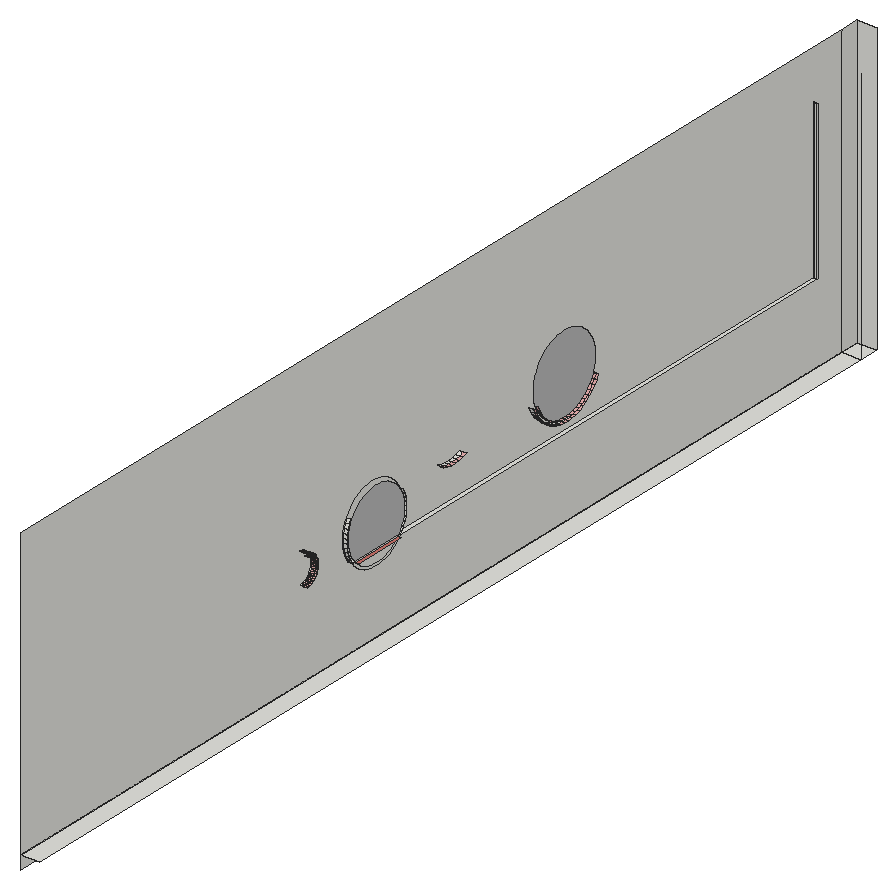
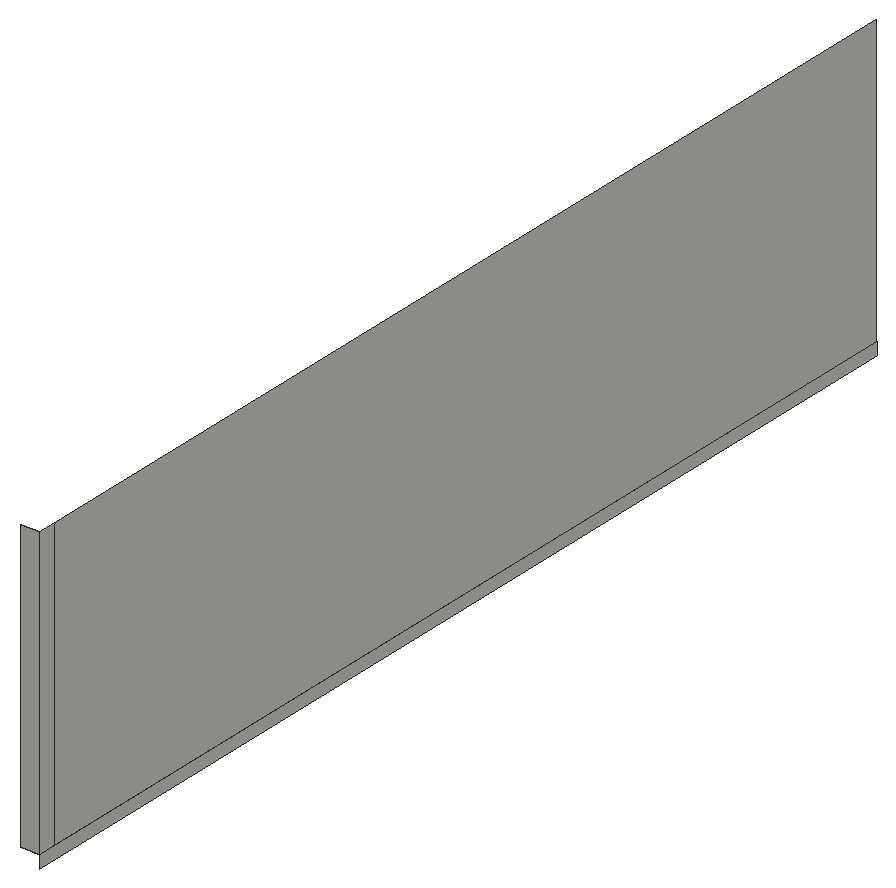
# SketchUp Ruby script. Lengths in inches.
U = 1.inch
M = Sketchup.active_model
def pt(a) = Geom::Point3d.new(a.map { |v| v * U })
def face(e, loops, mat)
  f = e.add_face(loops[0].map { |a| pt(a) })
  loops[1..].each { |l| e.add_face(l.map { |a| pt(a) }).erase! }
  f.material = f.back_material = mat if mat
  f
end
# faces: each face lists its corners as indices into pts; further lists are holes
def faces(e, pts, list, mat = nil) = list.each { |f| face(e, (f[0].is_a?(Array) ? f : [f]).map { |l| l.map { |i| pts[i] } }, mat) }
# xy, xz, yz: faces in a plane at the given z, y or x. An outline is a flat list of corners, or four numbers for a rectangle; further outlines are holes
def ring(l) = l.size == 4 ? [[l[0], l[1]], [l[2], l[1]], [l[2], l[3]], [l[0], l[3]]] : l.each_slice(2).to_a
def flat(e, list, mat, &to3) = list.each { |f| face(e, (f[0].is_a?(Array) ? f : [f]).map { |l| ring(l).map { |u, v| to3.(u, v) } }, mat) }
def xy(e, z, list, mat = nil) = flat(e, list, mat) { |x, y| [x, y, z] }
def xz(e, y, list, mat = nil) = flat(e, list, mat) { |x, z| [x, y, z] }
def yz(e, x, list, mat = nil) = flat(e, list, mat) { |y, z| [x, y, z] }
def lines(e, pts, list) = list.each { |a, b| e.add_line(pt(pts[a]), pt(pts[b])) }
# prism: a flat outline (further loops are holes) pulled along v
def prism(e, loops, v, mat = nil)
  f = face(e, loops, mat); d = Geom::Vector3d.new(v.map { |x| x * U })
  f.pushpull(f.normal.samedirection?(d) ? d.length : -d.length)
end
def box(e, o, s, mat = nil) = prism(e, [[o, [o[0] + s[0], o[1], o[2]], [o[0] + s[0], o[1] + s[1], o[2]], [o[0], o[1] + s[1], o[2]]]], [0, 0, s[2]], mat)
def at(x, y, z, deg = 0) = Geom::Transformation.translation(pt([x, y, z])) * Geom::Transformation.rotation(ORIGIN, Z_AXIS, deg.degrees)
def axes(o, x, y, z) = Geom::Transformation.new([*x, 0, *y, 0, *z, 0, *pt(o).to_a, 1])
def part(name) = M.definitions.add(name)
# library, detail: a bought-in or finely detailed component or shape, given as its bounding box
def library(name, o, s) = part(name).tap { |d| box(d.entities, o, s) }
def detail(e, o, s) = box(e.add_group.entities, o, s)
def put(e, d, t, mat = nil) = e.add_instance(d, t).tap { |i| i.material = mat if mat }
def group(e, t, mat = nil) = e.add_group.tap { |g| g.transformation = t; g.material = mat if mat }.entities
root = M.entities
M.materials.add("Generic").color = [224, 169, 169]
M.materials.add("[Mirror 01]").color = [185, 185, 185]
M.materials.add("[Wood Floor Dark]").color = [198, 114, 106]
xy(root,0,[[0,0.4375,9,481.125],[0,481.125,9,490.125]])
xy(root,46.5,[[9,181.21,10.6875,181.21,10.6875,196.98,9,198.375],[10.6875,196.98,10.6875,209.04,9,209.04,9,198.375],[9,209.04,10.6875,453.375],[9,453.375,10.6875,453.625]])
xy(root,46.5,[[10.6875,182.81,12.375,207.45]],"[Wood Floor Dark]")
xz(root,453.375,[[9,46.5,10.6875,120]])
xz(root,453.625,[[9,46.5,10.6875,120]])
xz(root,490.125,[[0,0,9,135.25]])
yz(root,0,[[0,-6,490.125,0],[0.4375,0,481.125,135.25],[481.125,0,490.125,135.25]])
yz(root,9,[[181.21,46.5,209.04,46.5,209.84,47.59,210.84,49.33,211.63,51.17,212.21,53.09,212.56,55.07,212.6875,57.07,212.58,59.07,212.25,61.05,211.7,62.97,210.93,64.82,209.95,66.58,208.78,68.2,207.4375,69.69,205.93,71.01,204.28,72.15,202.51,73.1,200.65,73.84,198.71,74.36,196.73,74.65,194.73,74.72,192.73,74.5625,190.76,74.18,188.85,73.57,187.02,72.74,185.3,71.72,183.7,70.5,182.26,69.11,180.98,67.57,179.89,65.89,178.99,64.1,178.31,62.21,177.84,60.26,177.6,58.27,177.59,56.27,177.81,54.27,178.25,52.32,178.91,50.42,179.79,48.62,180.86,46.93],[453.375,46.5,453.625,120]])
yz(root,10.6875,[[194.52,39.62,196.53,39.66,198.52,39.9375,200.46,40.4375,202.33,41.15,204.11,42.08,205.77,43.2,207.29,44.5,208.66,45.97,209.04,46.5,207.45,46.5,206.43,45.4,205.01,44.19,203.47,43.15,201.82,42.29,200.08,41.625,198.27,41.16,196.43,40.91,194.57,40.86,192.71,41.03,190.89,41.41,189.12,42,187.43,42.78,185.84,43.75,184.375,44.9,183.05,46.21,182.81,46.5,181.21,46.5,182.12,45.37,183.55,43.96,185.13,42.73,186.84,41.68,188.66,40.84,190.57,40.21,192.53,39.8],[194.57,40.86,196.43,40.91,198.27,41.16,200.08,41.625,201.82,42.29,203.47,43.15,205.01,44.19,206.43,45.4,207.45,46.5,182.81,46.5,183.05,46.21,184.375,44.9,185.84,43.75,187.43,42.78,189.12,42,190.89,41.41,192.71,41.03],[453.375,46.5,453.625,120]])
yz(root,10.6875,[[182.81,46.5,207.45,46.5,207.7,46.77,208.8,48.27,209.72,49.89,210.46,51.6,210.99,53.38,211.32,55.22,211.4375,57.07,211.34,58.93,211.04,60.77,210.52,62.5625,209.81,64.28,208.9,65.91,207.8125,67.42,206.5625,68.8,205.16,70.03,203.63,71.09,201.99,71.97,200.26,72.65,198.46,73.14,196.62,73.41,194.75,73.48,192.9,73.33,191.07,72.97,189.3,72.4,187.6,71.64,186,70.69,184.52,69.56,183.17,68.27,181.98,66.83,180.97,65.27,180.14,63.6,179.5,61.85,179.07,60.04,178.85,58.19,178.84,56.33,179.04,54.48,179.45,52.66,180.06,50.9,180.875,49.23,181.875,47.65],[305.93,53.75,307.99,53.95,310.02,54.375,311.98,55.03,313.86,55.9,315.62,56.99,317.25,58.26,318.72,59.72,320.02,61.33,321.12,63.08,322.02,64.94,322.7,66.9,323.15,68.92,323.375,70.97,323.36,73.04,323.11,75.1,322.62,77.11,321.91,79.05,320.98,80.9,319.85,82.64,318.53,84.23,317.03,85.66,315.38,86.91,313.6,87.96,311.71,88.81,309.74,89.43,307.71,89.83,305.64,89.99,303.58,89.91,301.53,89.6,299.53,89.06,297.61,88.29,295.79,87.3125,294.09,86.13,292.54,84.76,291.15,83.23,289.95,81.54,288.94,79.73,288.15,77.82,287.58,75.83,287.25,73.79,287.15,71.72,287.28,69.66,287.65,67.62,288.25,65.64,289.07,63.74,290.1,61.95,291.33,60.28,292.74,58.77,294.32,57.43,296.03,56.27,297.87,55.32,299.81,54.58,301.8125,54.07,303.86,53.8]],"[Mirror 01]")
p = [[10.6875,180.86,46.93],[10.6875,181.21,46.5],[9,181.21,46.5],[9,180.86,46.93],[10.6875,209.04,46.5],[10.6875,209.84,47.59],
  [9,209.84,47.59],[9,209.04,46.5],[10.6875,179.79,48.62],[9,179.79,48.62],[10.6875,210.84,49.33],[9,210.84,49.33],
  [10.6875,178.91,50.42],[9,178.91,50.42],[10.6875,152.83,49.33],[10.6875,153.61,49.5],[9,153.61,49.5],[9,152.83,49.33],
  [12.375,153.61,49.5],[12.375,152.83,49.33],[10.6875,211.63,51.17],[9,211.63,51.17],[10.6875,154.38,49.76],[9,154.38,49.76],
  [12.375,154.38,49.76],[10.6875,155.11,50.09],[9,155.11,50.09],[12.375,155.11,50.09],[10.6875,155.8,50.51],[9,155.8,50.51],
  [12.375,155.8,50.51],[10.6875,178.25,52.32],[9,178.25,52.32],[10.6875,156.44,51],[9,156.44,51],[12.375,156.44,51],
  [10.6875,153.22,50.95],[10.6875,152.59,50.8125],[12.375,152.59,50.8125],[12.375,153.22,50.95],[10.6875,153.83,51.15],[12.375,153.83,51.15],
  [10.6875,157.02,51.55],[9,157.02,51.55],[12.375,157.02,51.55],[10.6875,154.41,51.42],[12.375,154.41,51.42],[10.6875,212.21,53.09],
  [9,212.21,53.09],[10.6875,154.96,51.75],[12.375,154.96,51.75],[10.6875,157.54,52.17],[9,157.54,52.17],[12.375,157.54,52.17],
  [10.6875,155.47,52.14],[12.375,155.47,52.14],[10.6875,155.93,52.58],[12.375,155.93,52.58],[10.6875,157.99,52.84],[9,157.99,52.84],
  [12.375,157.99,52.84],[10.6875,303.74,52.28],[10.6875,305.99,52.23],[9,305.99,52.23],[9,303.74,52.28],[12,305.99,52.23],
  [12,303.74,52.28],[10.6875,308.22,52.44],[9,308.22,52.44],[12,308.22,52.44],[10.6875,177.81,54.27],[9,177.81,54.27],
  [10.6875,301.52,52.58],[9,301.52,52.58],[12,301.52,52.58],[10.6875,310.42,52.9],[9,310.42,52.9],[12,310.42,52.9],
  [10.6875,156.34,53.07],[12.375,156.34,53.07],[10.6875,299.35,53.13],[9,299.35,53.13],[12,299.35,53.13],[10.6875,158.36,53.56],
  [9,158.36,53.56],[12.375,158.36,53.56],[10.6875,312.54,53.61],[9,312.54,53.61],[12,312.54,53.61],[10.6875,156.7,53.6],
  [12.375,156.7,53.6],[10.6875,212.56,55.07],[9,212.56,55.07],[10.6875,297.25,53.93],[9,297.25,53.93],[12,297.25,53.93],
  [10.6875,156.99,54.17],[12.375,156.99,54.17],[10.6875,158.65,54.31],[9,158.65,54.31],[12.375,158.65,54.31],[10.6875,314.58,54.5625],
  [9,314.58,54.5625],[12,314.58,54.5625],[10.6875,303.86,53.8],[10.6875,301.8125,54.07],[12,301.8125,54.07],[12,303.86,53.8],
  [10.6875,305.93,53.75],[12,305.93,53.75],[10.6875,307.99,53.95],[12,307.99,53.95],[10.6875,295.26,54.96],[9,295.26,54.96],
  [12,295.26,54.96],[10.6875,310.02,54.375],[12,310.02,54.375],[10.6875,299.81,54.58],[12,299.81,54.58],[10.6875,157.22,54.77],
  [12.375,157.22,54.77],[10.6875,158.85,55.09],[9,158.85,55.09],[12.375,158.85,55.09],[10.6875,177.59,56.27],[9,177.59,56.27],
  [10.6875,311.98,55.03],[12,311.98,55.03],[10.6875,297.87,55.32],[12,297.87,55.32],[10.6875,316.49,55.74],[9,316.49,55.74],
  [12,316.49,55.74],[10.6875,157.38,55.39],[12.375,157.38,55.39],[10.6875,293.4,56.21],[9,293.4,56.21],[12,293.4,56.21],
  [10.6875,313.86,55.9],[12,313.86,55.9],[10.6875,158.97,55.88],[9,158.97,55.88],[12.375,158.97,55.88],[10.6875,212.6875,57.07],
  [9,212.6875,57.07],[10.6875,296.03,56.27],[12,296.03,56.27],[10.6875,157.48,56.02],[12.375,157.48,56.02],[10.6875,318.25,57.12],
  [9,318.25,57.12],[12,318.25,57.12],[10.6875,159,56.6875],[9,159,56.6875],[12.375,159,56.6875],[10.6875,315.62,56.99],
  [12,315.62,56.99],[10.6875,157.5,56.66],[12.375,157.5,56.66],[10.6875,291.69,57.67],[9,291.69,57.67],[12,291.69,57.67],
  [10.6875,177.6,58.27],[9,177.6,58.27],[10.6875,294.32,57.43],[12,294.32,57.43],[10.6875,157.45,57.3],[12.375,157.45,57.3],
  [10.6875,158.94,57.49],[9,158.94,57.49],[12.375,158.94,57.49],[10.6875,317.25,58.26],[12,317.25,58.26],[10.6875,212.58,59.07],
  [9,212.58,59.07],[10.6875,319.85,58.7],[9,319.85,58.7],[12,319.85,58.7],[10.6875,157.34,57.93],[12.375,157.34,57.93],
  [10.6875,292.74,58.77],[12,292.74,58.77],[10.6875,158.79,58.28],[9,158.79,58.28],[12.375,158.79,58.28],[10.6875,290.16,59.31],
  [9,290.16,59.31],[12,290.16,59.31],[10.6875,157.15,58.54],[12.375,157.15,58.54],[10.6875,158.56,59.06],[9,158.56,59.06],
  [12.375,158.56,59.06],[10.6875,177.84,60.26],[9,177.84,60.26],[10.6875,318.72,59.72],[12,318.72,59.72],[10.6875,156.9,59.13],
  [12.375,156.9,59.13],[10.6875,321.26,60.44],[9,321.26,60.44],[12,321.26,60.44],[10.6875,291.33,60.28],[12,291.33,60.28],
  [10.6875,156.58,59.6875],[12.375,156.58,59.6875],[10.6875,158.24,59.8],[9,158.24,59.8],[12.375,158.24,59.8],[10.6875,212.25,61.05],
  [9,212.25,61.05],[10.6875,288.83,61.11],[9,288.83,61.11],[12,288.83,61.11],[10.6875,156.21,60.21],[12.375,156.21,60.21],
  [10.6875,320.02,61.33],[12,320.02,61.33],[10.6875,157.85,60.5],[9,157.85,60.5],[12.375,157.85,60.5],[10.6875,155.78,60.68],
  [12.375,155.78,60.68],[10.6875,178.31,62.21],[9,178.31,62.21],[10.6875,290.1,61.95],[12,290.1,61.95],[10.6875,322.45,62.34],
  [9,322.45,62.34],[12,322.45,62.34],[10.6875,157.375,61.15],[9,157.375,61.15],[12.375,157.375,61.15],[10.6875,155.3,61.11],
  [12.375,155.3,61.11],[10.6875,211.7,62.97],[9,211.7,62.97],[10.6875,154.78,61.48],[12.375,154.78,61.48],[10.6875,287.71,63.06],
  [9,287.71,63.06],[12,287.71,63.06],[10.6875,156.84,61.75],[9,156.84,61.75],[12.375,156.84,61.75],[10.6875,321.12,63.08],
  [12,321.12,63.08],[10.6875,154.22,61.79],[12.375,154.22,61.79],[10.6875,156.23,62.28],[9,156.23,62.28],[12.375,156.23,62.28],
  [10.6875,153.63,62.04],[12.375,153.63,62.04],[10.6875,289.07,63.74],[12,289.07,63.74],[10.6875,153.01,62.22],[12.375,153.01,62.22],
  [10.6875,178.99,64.1],[9,178.99,64.1],[10.6875,155.58,62.75],[9,155.58,62.75],[12.375,155.58,62.75],[10.6875,323.43,64.36],
  [9,323.43,64.36],[12,323.43,64.36],[10.6875,154.87,63.14],[9,154.87,63.14],[12.375,154.87,63.14],[10.6875,210.93,64.82],
  [9,210.93,64.82],[10.6875,154.13,63.45],[9,154.13,63.45],[12.375,154.13,63.45],[10.6875,286.82,65.12],[9,286.82,65.12],
  [12,286.82,65.12],[10.6875,322.02,64.94],[12,322.02,64.94],[10.6875,153.35,63.67],[9,153.35,63.67],[12.375,153.35,63.67],
  [10.6875,235.21,63.91],[10.6875,237.4,63.61],[9,237.4,63.61],[9,235.21,63.91],[12.1875,237.4,63.61],[12.1875,235.21,63.91],
  [10.6875,239.61,63.57],[9,239.61,63.57],[12.1875,239.61,63.57],[10.6875,241.81,63.77],[9,241.81,63.77],[12.1875,241.81,63.77],
  [10.6875,152.5625,63.81],[9,152.5625,63.81],[12.375,152.5625,63.81],[10.6875,288.25,65.64],[12,288.25,65.64],[10.6875,243.97,64.23],
  [9,243.97,64.23],[12.1875,243.97,64.23],[10.6875,233.07,64.45],[9,233.07,64.45],[12.1875,233.07,64.45],[10.6875,179.89,65.89],
  [9,179.89,65.89],[10.6875,246.06,64.93],[9,246.06,64.93],[12.1875,246.06,64.93],[9,481.125,0],[9,481.125,120]]
faces(root,p,[[0,1,2,3],[4,5,6,7],[8,0,3,9],[5,10,11,6],[12,8,9,13],[14,15,16,17],[10,20,21,11],[15,22,23,16],
  [22,25,26,23],[25,28,29,26],[31,12,13,32],[28,33,34,29],[33,42,43,34],[20,47,48,21],[42,51,52,43],[51,58,59,52],
  [61,62,63,64],[62,67,68,63],[70,31,32,71],[72,61,64,73],[67,75,76,68],[80,72,73,81],[58,83,84,59],[75,86,87,76],
  [47,91,92,48],[93,80,81,94],[83,98,99,84],[86,101,102,87],[112,93,94,113],[98,121,122,99],[124,70,71,125],[101,130,131,102],
  [135,112,113,136],[121,140,141,122],[91,143,144,92],[130,149,150,131],[140,152,153,141],[159,135,136,160],[162,124,125,163],[152,168,169,153],
  [143,173,174,144],[149,175,176,150],[168,182,183,169],[185,159,160,186],[182,190,191,183],[193,162,163,194],[175,199,200,176],[190,206,207,191],
  [173,209,210,174],[211,185,186,212],[206,218,219,207],[223,193,194,224],[199,227,228,200],[218,230,231,219],[209,235,236,210],[239,211,212,240],
  [230,242,243,231],[242,249,250,243],[258,223,224,259],[249,260,261,250],[227,263,264,228],[260,266,267,261],[235,269,270,236],[266,271,272,267],
  [274,239,240,275],[271,279,280,272],[282,283,284,285],[283,288,289,284],[288,291,292,289],[279,294,295,280],[291,299,300,292],[302,282,285,303],
  [305,258,259,306],[299,307,308,300]])
faces(root,p,[[14,15,18,19],[15,22,24,18],[22,25,27,24],[25,28,30,27],[28,33,35,30],[36,37,38,39],[40,36,39,41],[33,42,44,35],
  [45,40,41,46],[49,45,46,50],[42,51,53,44],[54,49,50,55],[56,54,55,57],[51,58,60,53],[61,62,65,66],[62,67,69,65],
  [72,61,66,74],[67,75,77,69],[78,56,57,79],[80,72,74,82],[58,83,85,60],[75,86,88,77],[89,78,79,90],[93,80,82,95],
  [96,89,90,97],[83,98,100,85],[86,101,103,88],[104,105,106,107],[108,104,107,109],[110,108,109,111],[112,93,95,114],[115,110,111,116],
  [105,117,118,106],[119,96,97,120],[98,121,123,100],[126,115,116,127],[117,128,129,118],[101,130,132,103],[133,119,120,134],[135,112,114,137],
  [138,126,127,139],[121,140,142,123],[128,145,146,129],[147,133,134,148],[130,149,151,132],[140,152,154,142],[155,138,139,156],[157,147,148,158],
  [159,135,137,161],[145,164,165,146],[166,157,158,167],[152,168,170,154],[171,155,156,172],[149,175,177,151],[178,166,167,179],[164,180,181,165],
  [168,182,184,170],[185,159,161,187],[188,178,179,189],[182,190,192,184],[195,171,172,196],[197,188,189,198],[175,199,201,177],[180,202,203,181],
  [204,197,198,205],[190,206,208,192],[211,185,187,213],[214,204,205,215],[216,195,196,217],[206,218,220,208],[221,214,215,222],[202,225,226,203],
  [199,227,229,201],[218,230,232,220],[233,221,222,234],[237,233,234,238],[239,211,213,241],[230,242,244,232],[245,216,217,246],[247,237,238,248],
  [242,249,251,244],[252,247,248,253],[225,254,255,226],[256,252,253,257],[249,260,262,251],[227,263,265,229],[260,266,268,262],[266,271,273,268],
  [274,239,241,276],[277,245,246,278],[271,279,281,273],[282,283,286,287],[283,288,290,286],[288,291,293,290],[279,294,296,281],[254,297,298,255],
  [291,299,301,293],[302,282,287,304],[299,307,309,301]],"Generic")
lines(root,p,[[310,311]])
